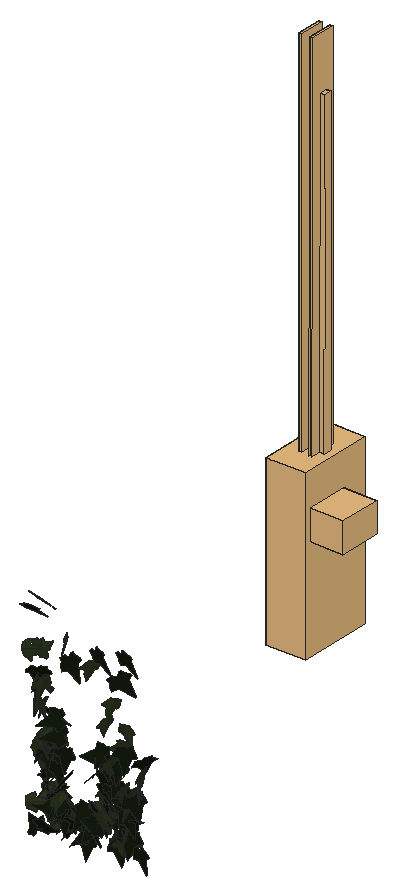
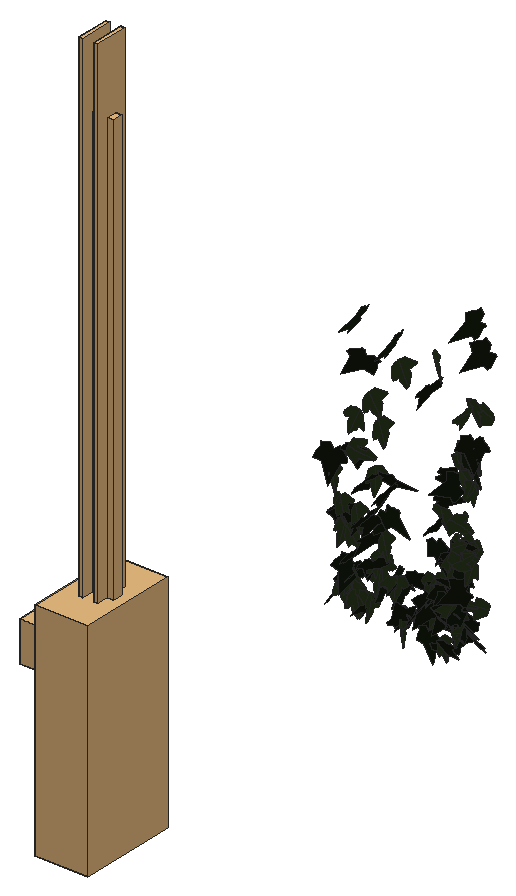
# SketchUp Ruby script. Lengths in inches.
U = 1.inch
M = Sketchup.active_model
def pt(a) = Geom::Point3d.new(a.map { |v| v * U })
def face(e, loops, mat)
  f = e.add_face(loops[0].map { |a| pt(a) })
  loops[1..].each { |l| e.add_face(l.map { |a| pt(a) }).erase! }
  f.material = f.back_material = mat if mat
  f
end
# faces: each face lists its corners as indices into pts; further lists are holes
def faces(e, pts, list, mat = nil) = list.each { |f| face(e, (f[0].is_a?(Array) ? f : [f]).map { |l| l.map { |i| pts[i] } }, mat) }
# xy, xz, yz: faces in a plane at the given z, y or x. An outline is a flat list of corners, or four numbers for a rectangle; further outlines are holes
def ring(l) = l.size == 4 ? [[l[0], l[1]], [l[2], l[1]], [l[2], l[3]], [l[0], l[3]]] : l.each_slice(2).to_a
def flat(e, list, mat, &to3) = list.each { |f| face(e, (f[0].is_a?(Array) ? f : [f]).map { |l| ring(l).map { |u, v| to3.(u, v) } }, mat) }
def xy(e, z, list, mat = nil) = flat(e, list, mat) { |x, y| [x, y, z] }
def xz(e, y, list, mat = nil) = flat(e, list, mat) { |x, z| [x, y, z] }
def yz(e, x, list, mat = nil) = flat(e, list, mat) { |y, z| [x, y, z] }
def lines(e, pts, list) = list.each { |a, b| e.add_line(pt(pts[a]), pt(pts[b])) }
# prism: a flat outline (further loops are holes) pulled along v
def prism(e, loops, v, mat = nil)
  f = face(e, loops, mat); d = Geom::Vector3d.new(v.map { |x| x * U })
  f.pushpull(f.normal.samedirection?(d) ? d.length : -d.length)
end
def box(e, o, s, mat = nil) = prism(e, [[o, [o[0] + s[0], o[1], o[2]], [o[0] + s[0], o[1] + s[1], o[2]], [o[0], o[1] + s[1], o[2]]]], [0, 0, s[2]], mat)
def at(x, y, z, deg = 0) = Geom::Transformation.translation(pt([x, y, z])) * Geom::Transformation.rotation(ORIGIN, Z_AXIS, deg.degrees)
def axes(o, x, y, z) = Geom::Transformation.new([*x, 0, *y, 0, *z, 0, *pt(o).to_a, 1])
def part(name) = M.definitions.add(name)
# library, detail: a bought-in or finely detailed component or shape, given as its bounding box
def library(name, o, s) = part(name).tap { |d| box(d.entities, o, s) }
def detail(e, o, s) = box(e.add_group.entities, o, s)
def put(e, d, t, mat = nil) = e.add_instance(d, t).tap { |i| i.material = mat if mat }
def group(e, t, mat = nil) = e.add_group.tap { |g| g.transformation = t; g.material = mat if mat }.entities
root = M.entities
M.materials.add("Glass Rail Metal").color = [192, 192, 192]
M.materials.add("[Translucent Glass Tinted]").color = [8, 201, 241]
M.materials["[Translucent Glass Tinted]"].alpha = 0.48
M.materials.add("efeu1").color = [18, 25, 13]
M.materials.add("efeu2").color = [43, 57, 29]
c1 = part("ivyleaf_9")
p = [[1.54,2.16,1.25],[1.36,2.04,1.19],[-0.21,0.99,0.68],[-0.71,1.11,0.82],[-0.85,0.86,0.67],[-0.8,0.17,0.21],
  [-0.9,-0.01,0.1],[-0.67,-0.16,-0.02],[-0.08,-0.08,-0.05],[-0.03,-0.6,-0.4],[0.65,-0.88,-0.66],[0.83,-0.6,-0.49],
  [1.29,-0.42,-0.43],[1.8125,-0.07,-0.26],[1.21,0.44,0.15]]
faces(c1.entities,p,[[0,1,2,3,4,5,6,7,8,9,10,11,12,13,14]],"efeu1")
c2 = part("ivyleaf_10")
p = [[0,0.5,-0.03],[-0.0625,2.02,-0.43],[-0.19,2.01,-0.46],[-0.54,1.05,-0.29],[-0.52,0.625,-0.18],[-0.83,0.76,-0.28],
  [-1.16,0.64,-0.33],[-1.15,0.33,-0.24],[-0.77,-0.39,0.02],[-0.3,-0.51,0.16],[0.04,-0.48,0.23],[-0.02,2.01,-0.4375],
  [-0.06,2.01,-0.43],[0.04,-0.49,0.23],[0.67,-0.49,0.14],[1.38,0.36,-0.2],[1.375,0.51,-0.24],[0.81,0.65,-0.19],
  [0.62,0.59,-0.15],[0.6,1.09,-0.28],[0.5,1.23,-0.31]]
faces(c2.entities,p,[[0,1,2,3,4,5,6,7,8,9,10],[11,12,0,13,14,15,16,17,18,19,20]],"efeu2")
c3 = library("glass bracket3",[-2.83,-0.98,-1],[3.67,3.29,2])
c4 = library("Group\#46",[0,0,0],[50.8,6,878.92])
c5 = library("Group\#15",[0.69,0,0.79],[0.62,1.89,30.3])
c6 = library("Group\#43",[0,0,0],[50.8,6,878.92])
c7 = library("Group\#53",[0,0,0],[3.15,5.91,11.14])
put(root,c1,axes([518.76,128.71,270.52],[0.73335,-0.82739,-0.07933],[0.07062,0.16744,-1.09346],[0.82818,0.71837,0.16349]))
put(root,c1,axes([508.96,129.22,258.32],[-0.73907,-0.28461,0.64117],[-0.60461,-0.2589,-0.77055],[0.41505,-0.88394,0.01925]))
put(root,c1,axes([505.71,128.29,274.43],[1.10412,-0.17355,0.00871],[0.04756,0.24793,-1.08883],[0.16713,1.07596,0.2523]))
put(root,c2,axes([513.88,129,267.48],[-0.28227,-1.01753,0.27722],[-0.03621,-0.27746,-1.05527],[1.05399,-0.28204,0.03799]))
put(root,c2,axes([516.99,128.65,255.53],[-0.22277,-1.0028,-0.22556],[0.03318,0.22366,-1.02713],[1.02732,-0.22468,-0.01574]))
put(root,c2,axes([509.16,128.75,248.03],[0.33895,0.95653,-0.16425],[-0.20094,-0.10349,-1.03639],[-1.02758,0.33575,0.14849]))
put(root,c1,axes([509.7,129.3,247.28],[-0.88288,-0.4898,0.19327],[-0.14417,-0.13829,-0.98979],[0.5471,-0.82686,0.05106]))
put(root,c1,axes([509.53,129.25,245.82],[0.01955,-0.95938,0.0947],[0.00483,-0.09099,-0.99793],[1.04078,0.01845,0.00285]))
put(root,c2,axes([510.04,128.89,269.49],[0.60989,-0.91075,-0.05301],[-0.01169,0.05595,-1.09589],[0.91222,0.60963,0.02139]))
put(root,c1,axes([506.24,128.73,243.21],[0.53244,-0.18494,0.76957],[0.78135,-0.16562,-0.54434],[0.26085,0.87359,0.05971]))
put(root,c1,axes([509.93,128.92,246.58],[-0.91388,0.50314,-0.2297],[0.19303,-0.13147,-1.02361],[-0.56118,-0.8646,0.02197]))
put(root,c2,axes([516.17,129.01,260.7],[-0.07613,-1.0616,0.10446],[0.01558,-0.10582,-1.06408],[1.06661,-0.07423,0.02299]))
put(root,c1,axes([514.6875,128.83,269.47],[0.75757,-0.77519,-0.19052],[-0.05686,0.20959,-1.07887],[0.79623,0.75251,0.10423]))
put(root,c2,axes([519.01,128.84,260.71],[-1.0052,0.2156,-0.32106],[0.29146,-0.16535,-1.02357],[-0.25419,-1.04219,0.09598]))
put(root,c1,axes([514.1,129.59,245.81],[-0.65738,-0.79377,0.25529],[-0.12052,-0.23122,-1.02927],[0.82505,-0.66623,0.05306]))
put(root,c2,axes([504.96,128.62,246.02],[0.22266,-0.0161,-0.94755],[0.94219,0.27331,0.20028],[0.28427,-0.89326,0.07836]))
put(root,c2,axes([506.76,128.87,254.4],[-0.65316,0.72386,-0.13088],[0.08258,-0.1001,-0.98097],[-0.78919,-0.60957,0.00568]))
put(root,c2,axes([516.92,129.34,263.35],[-0.3207,-0.9462,0.41234],[-0.01464,-0.42757,-0.99254],[1.03204,-0.30009,0.11405]))
put(root,c2,axes([515.79,128.93,247.58],[-0.99595,0.08341,-0.22059],[0.21073,-0.11506,-0.99493],[-0.10588,-1.01357,0.09479]))
put(root,c1,axes([515.46,129.13,255.62],[-0.78114,0.26971,0.6486],[-0.66455,0.03054,-0.81305],[-0.22759,-1.01486,0.1479]))
put(root,c1,axes([515.29,129.05,251.34],[0.84604,-0.67912,0.01835],[0.01525,-0.01032,-1.08489],[0.6792,0.84618,0.0015]))
put(root,c1,axes([515.52,128.67,253.86],[0.75836,-0.50956,-0.60101],[-0.37926,0.49511,-0.89833],[0.69067,0.83138,0.16662]))
put(root,c1,axes([509.02,129.59,255.82],[-0.62408,-0.18442,0.76326],[-0.71289,-0.32869,-0.62642],[0.39962,-0.87436,0.0745]))
put(root,c1,axes([509.99,128.8125,250.79],[-0.36749,0.91471,-0.15469],[0.05626,-0.13932,-1.01499],[-0.99928,-0.34424,-0.00026]))
put(root,c1,axes([518.77,129.32,257.58],[-0.73748,-0.49811,-0.58047],[0.48116,0.3247,-0.88994],[0.5946,-0.88056,0.0002]))
put(root,c2,axes([503.87,129.2,266.02],[0.32529,-0.18619,-0.9766],[0.97258,-0.27888,0.35791],[-0.35078,-0.9459,0.08671]))
put(root,c1,axes([507.17,128.55,248.64],[-0.15352,0.88052,0.29835],[-0.03681,0.28506,-0.92752],[-0.99948,-0.14575,-0.01167]))
put(root,c1,axes([513.19,129.57,244.82],[0.48168,-0.76677,0.5409],[0.38793,-0.3909,-0.89958],[0.85442,0.60974,0.1035]))
put(root,c1,axes([512.57,129.75,247.12],[-0.81766,-0.66586,0.01126],[-0.00826,-0.00769,-1.05448],[0.66591,-0.8177,0.00074]))
put(root,c2,axes([506.3,129.7,259.64],[0.28617,-0.79006,0.53749],[0.18463,-0.48776,-0.86662],[1.00275,0.31528,0.00617]))
put(root,c1,axes([517.8,129.0625,267.0625],[-0.10809,-0.35572,-1.02995],[0.5617,0.8687,-0.35898],[0.93372,-0.56377,0.09672]))
put(root,c1,axes([505.76,128.83,242.59],[-0.03602,0.49112,0.79904],[-0.60292,0.5969,-0.42202],[-0.77868,-0.48489,0.2898]))
put(root,c2,axes([506.15,129.59,262.2],[-0.13474,-1.03985,0.2075],[0.02286,-0.21196,-1.0474],[1.0601,-0.1276,0.04895]))
put(root,c1,axes([504.26,128.85,272.14],[1.07639,0.14162,0.11916],[0.09234,0.19902,-1.02933],[-0.17372,0.98328,0.19118]))
put(root,c1,axes([519.84,129.47,251.38],[-0.26919,-0.81765,-0.59146],[0.24318,0.54154,-0.85932],[0.97941,-0.3592,0.0508]))
put(root,c1,axes([510.23,129.37,266.84],[0.27012,-0.92167,-0.51108],[-0.10495,0.50145,-0.95977],[1.04864,0.2876,0.03559]))
put(root,c1,axes([509.58,128.91,245.02],[0.93279,0.51284,-0.07704],[-0.07071,-0.03482,-1.04465],[-0.55513,0.86617,0.00361]))
put(root,c2,axes([518.68,129.52,257.74],[0.30599,0.17713,-1.00278],[-1.01535,-0.02668,-0.31454],[-0.07756,1.04809,0.16147]))
put(root,c1,axes([517.2,130.09,255.01],[-0.14461,-1.02549,0.18647],[-0.00133,-0.18807,-1.03535],[1.04231,-0.14252,0.02455]))
put(root,c1,axes([507.49,129.92,245.77],[-0.6914,0.09464,0.66822],[-0.6891,-0.25994,-0.62134],[0.13084,-0.86896,0.25865]))
put(root,c2,axes([510.15,129.42,247.38],[-0.93441,0.47797,-0.06146],[0.06324,-0.01621,-1.02788],[-0.51628,-0.86706,-0.01467]))
put(root,c1,axes([509.02,130.23,253.75],[-0.02735,-1.0253,0.17872],[0.02701,-0.17942,-1.02519],[1.04041,-0.0223,0.03131]))
put(root,c2,axes([508.98,129.22,244.85],[0.63698,0.60096,0.5701],[0.14931,0.5932,-0.83103],[-0.8657,0.54449,0.27615]))
put(root,c2,axes([505.37,129.62,266.9],[0.81921,-0.44131,-0.45466],[-0.37676,0.26829,-0.91115],[0.5551,0.83337,0.05256]))
put(root,c1,axes([507.82,130.125,251.24],[0.18293,-0.91464,0.06599],[0.00096,-0.06436,-0.96733],[0.99018,0.16904,-0.01126]))
put(root,c2,axes([504.79,129.98,259.35],[-0.14666,0.82408,-0.47353],[-0.0054,-0.46065,-0.86554],[-1.01681,-0.11642,0.0729]))
put(root,c1,axes([512.28,130.27,243.04],[-0.01752,-0.99155,0.12454],[-0.02793,-0.12402,-0.99138],[0.99895,-0.02086,-0.02553]))
put(root,c2,axes([518.6,130.21,249.74],[0.15325,-0.92037,0.46601],[0.11957,-0.45211,-0.93222],[1.02467,0.19041,0.03908]))
put(root,c2,axes([520.89,129.81,254.97],[0.21102,-1.0348,-0.11686],[0.0168,0.12261,-1.05532],[1.04125,0.20773,0.04071]))
put(root,c2,axes([518.05,129.93,251.87],[0.08153,-1.04614,-0.0366],[0.00107,0.0368,-1.0493],[1.04678,0.08144,0.00392]))
put(root,c1,axes([512.48,130.18,243.78],[-0.9715,0.24702,-0.02149],[-0.03589,-0.22609,-0.97616],[-0.24534,-0.94507,0.22791]))
put(root,c2,axes([504.76,129.91,262.35],[0.51133,-0.83041,-0.17849],[-0.10616,0.14149,-0.99401],[0.90963,0.48331,-0.01568]))
put(root,c1,axes([514.71,130.23,254.89],[0.20272,-1.02413,-0.08631],[-0.0045,0.08709,-1.04393],[1.02775,0.20238,0.01245]))
put(root,c2,axes([519.66,130.07,252.21],[0.04143,-1.05163,0.02218],[-0.03348,-0.0235,-1.05188],[1.05133,0.04069,-0.03437]))
put(root,c1,axes([518.72,130.37,245.57],[-0.42712,-0.89986,-0.20001],[0.05613,0.19464,-0.99557],[0.92011,-0.42959,-0.03211]))
put(root,c2,axes([515.48,130.01,247.48],[-0.86181,-0.5295,0.15653],[-0.13407,-0.0808,-1.01148],[0.53563,-0.87218,-0.00132]))
put(root,c2,axes([508.29,130.1,255.33],[1.01895,-0.12137,-0.02746],[-0.02697,0.01282,-0.98925],[0.13141,0.94376,0.0099]))
put(root,c1,axes([515.43,130.74,247.52],[0.0813,-0.77395,0.66392],[0.07404,-0.65978,-0.7782],[1.017,0.10991,0.00358]))
put(root,c2,axes([507.6,129.92,244.93],[0.52833,-0.65279,-0.42046],[-0.21607,0.35444,-0.84696],[0.80062,0.52642,0.04888]))
put(root,c1,axes([506.73,129.9,258.26],[0.95307,-0.17529,0.37982],[0.39869,-0.01252,-0.93393],[0.18017,0.95497,0.05748]))
put(root,c1,axes([517.07,130.17,251.57],[0.32929,-0.91008,-0.37758],[-0.05653,0.38001,-0.96522],[0.98367,0.32649,0.07093]))
put(root,c1,axes([520.97,129.63,256.75],[0.38021,0.99082,-0.14473],[-0.0394,-0.13989,-1.06118],[-1.00055,0.38202,-0.01321]))
put(root,c1,axes([512.32,130.12,243.88],[-0.81306,0.58648,0.01633],[-0.04904,-0.04012,-1.00064],[-0.58465,-0.81224,0.06122]))
put(root,c1,axes([514.32,130.28,253.04],[-0.65313,0.71302,-0.37936],[0.02187,-0.47209,-0.92496],[-0.80737,-0.58959,0.28184]))
put(root,c1,axes([507,130.64,251.78],[-0.54028,-0.79789,-0.02459],[0.01111,0.02146,-0.97942],[0.86203,-0.50036,-0.00279]))
put(root,c1,axes([519.375,130.4,251.21],[-0.66665,-0.45262,-0.66713],[0.57166,0.345,-0.80532],[0.56845,-0.87776,0.02749]))
put(root,c2,axes([504.79,130.33,258.76],[-0.70573,0.3914,-0.61027],[0.50647,-0.35645,-0.79037],[-0.56904,-0.80267,0.0534]))
put(root,c1,axes([504.91,129.96,263.36],[0.51956,0.72287,-0.45402],[-0.27846,-0.3527,-0.90287],[-0.86847,0.54554,0.01787]))
put(root,c2,axes([520,130.14,252.39],[-0.77347,0.70826,0.12326],[-0.20972,-0.04913,-1.03377],[-0.68763,-0.78169,0.17665]))
put(root,c1,axes([505.47,130.1,261.54],[-0.57354,0.80182,0.02035],[-0.01007,0.01729,-1.0002],[-0.86616,-0.53114,-0.00184]))
put(root,c2,axes([518.22,130.06,245.77],[0.28283,-0.85179,-0.48721],[0.10749,0.53088,-0.86575],[0.97538,0.18849,0.23668]))
put(root,c1,axes([509.66,129.875,245.41],[0.90681,0.46455,0.0102],[0.0012,0.01824,-0.99783],[-0.50182,0.8395,0.01604]))
put(root,c2,axes([504.72,130.15,252.16],[-0.43262,-0.24929,0.86718],[0.76985,0.43264,0.49066],[-0.53924,0.81765,0.00476]))
put(root,c2,axes([518.46,130.76,245.47],[-0.69874,-0.6287,0.40681],[-0.03492,-0.52844,-0.87666],[0.74803,-0.61195,0.33907]))
put(root,c2,axes([514.56,130.49,250.4],[0.09787,-1.03114,-0.01242],[-0.00181,0.01231,-1.03577],[1.03121,0.09788,-0.00064]))
put(root,c1,axes([519.79,130.7,243.58],[0.38989,-0.93612,0.00333],[-0.01495,-0.00984,-1.01392],[0.93601,0.38978,-0.01758]))
put(root,c2,axes([504.72,130.49,253.6],[0.5534,0.00055,0.83687],[0.86901,0.00988,-0.53288],[-0.00932,0.95393,0.00504]))
put(root,c2,axes([505.92,130.52,261.125],[-0.9754,0.07278,0.28799],[0.29814,-0.0217,0.94232],[0.08202,0.94439,-0.00054]))
put(root,c1,axes([515.68,130.3125,252.15],[0.21412,-0.80032,-0.63154],[-0.13394,0.61764,-0.82812],[1.01066,0.25141,0.02405]))
put(root,c1,axes([517.79,130.74,245.9],[0.27451,-0.98439,-0.09733],[-0.00618,0.0993,-1.02174],[0.98917,0.27381,0.02062]))
put(root,c1,axes([517.85,130.61,248.06],[0.26684,-0.95174,-0.29866],[-0.01607,0.30502,-0.98637],[0.99738,0.25955,0.06401]))
put(root,c2,axes([518.1,130.72,245.27],[-0.13822,0.8933,-0.48133],[-0.12004,-0.49676,-0.88747],[-1.0076,-0.06336,0.17176]))
put(root,c1,axes([505.68,130.88,253.27],[-0.90194,-0.38212,-0.11304],[0.12287,0.01238,-0.95441],[0.41109,-0.84208,0.03726]))
put(root,c1,axes([505.5625,131,243.18],[0.2356,-0.46354,0.79773],[0.3846,-0.67962,-0.53246],[0.88824,0.41722,0.01896]))
put(root,c1,axes([514.03,131.14,245.43],[0.152,-0.74203,0.67043],[0.26904,-0.62278,-0.7503],[0.96317,0.29106,0.10378]))
put(root,c1,axes([507.8,130.19,247.3],[0.5773,0.69456,-0.26873],[-0.16023,-0.21185,-0.91143],[-0.78415,0.55463,-0.0116]))
put(root,c1,axes([515.51,130.79,247.96],[-0.2666,-0.85622,-0.49563],[0.21267,0.45171,-0.89474],[0.96619,-0.33568,0.06019]))
put(root,c2,axes([519.1,130.3125,250.38],[-0.30876,-0.87098,-0.4879],[0.16206,0.46019,-0.92409],[0.98508,-0.34871,-0.0009]))
put(root,c2,axes([518.69,130.8,244.63],[-0.74369,-0.67808,0.16239],[-0.02619,-0.21009,-0.99721],[0.69676,-0.73165,0.13585]))
put(root,c1,axes([510.52,130.7,244.71],[0.5289,-0.81515,-0.27055],[-0.07967,0.26981,-0.96863],[0.85517,0.52928,0.07709]))
put(root,c1,axes([512.78,130.98,247.1],[0.58204,-0.79216,0.25625],[0.15376,-0.205,-0.983],[0.81826,0.602,0.00245]))
put(root,c1,axes([516.29,131.01,243.42],[0.05873,-0.99008,-0.17126],[0.0295,0.17318,-0.99104],[1.00435,0.05281,0.03913]))
put(root,c1,axes([505.875,131.23,246.56],[0.78542,-0.50554,-0.22986],[0.18898,-0.13547,0.92105],[-0.56512,-0.74792,-0.01146]))
put(root,c2,axes([517.3,130.91,243.86],[-0.66233,-0.76235,0.1255],[0.0534,-0.21008,-0.9943],[0.77077,-0.64054,0.17673]))
put(root,c2,axes([515.23,130.49,246.71],[-0.83649,0.5067,0.28852],[-0.2507,0.14299,-0.97796],[-0.52644,-0.87322,0.00728]))
put(root,c1,axes([515.64,130.64,250.4],[0.20452,-0.74911,-0.68119],[0.08285,0.705,-0.75042],[1.00912,0.09394,0.19967]))
put(root,c2,axes([506.89,130.76,251.54],[-0.09137,0.9309,-0.12397],[-0.00036,-0.11972,-0.97206],[-1.01358,-0.08387,0.01152]))
put(root,c2,axes([504.57,130.67,251.25],[-0.95363,0.32095,-0.05913],[0.06595,0.0016,-0.97681],[-0.34579,-0.88482,-0.02322]))
put(root,c2,axes([517.29,130.91,244.13],[-0.32522,-0.96677,0.02313],[-0.00756,-0.02186,-1.02],[0.96701,-0.3253,-0.00019]))
put(root,c2,axes([506.05,131.2,255.49],[0.40094,0.42435,-0.74963],[-0.72126,-0.32442,-0.55636],[-0.54389,0.74304,0.1852]))
put(root,c2,axes([505.47,130.23,266.04],[0.29521,0.03463,-0.96041],[0.23469,0.93361,0.1033],[0.97007,-0.23641,0.26728]))
put(root,c1,axes([509.38,130.65,242.88],[-0.1698,0.93445,0.0318],[0.00577,0.03191,-0.98543],[-1.00973,-0.15696,-0.01098]))
put(root,c2,axes([515.74,130.8,244.12],[0.08287,-0.88455,-0.49433],[0.06391,0.49955,-0.88318],[1.01128,0.04091,0.09633]))
put(root,c2,axes([517.61,130.82,245.37],[0.18304,-0.0135,1.0075],[-0.98697,0.20373,0.18204],[-0.20283,-1.00352,0.02341]))
put(root,c2,axes([505.6,131.47,251.61],[0.42278,0.40341,0.75194],[-0.54032,-0.52199,0.5846],[0.71248,-0.63524,-0.00286]))
put(root,c2,axes([512.77,131.05,247.14],[0.66969,0.75499,0.11689],[-0.06111,0.20788,-0.99257],[-0.76153,0.64725,0.18245]))
put(root,c1,axes([518.03,130.66,246.87],[0.62213,0.82066,-0.01773],[-0.1177,0.06716,-1.02102],[-0.81237,0.61874,0.13435]))
put(root,c1,axes([507.09,130.91,247.26],[0.00462,0.893,-0.03847],[-0.00241,-0.03698,-0.92873],[-0.96526,0.00436,0.00214]))
put(root,c2,axes([505.85,131.36,246.4],[0.91693,0.33119,-0.02119],[-0.01948,-0.00981,-0.94777],[-0.35783,0.8492,-0.00269]))
put(root,c2,axes([506.07,131.14,252.92],[-0.4676,0.21768,-0.8078],[-0.71953,0.40051,0.50296],[0.49117,0.79395,-0.03223]))
put(root,c2,axes([507.1,131.64,243.12],[0.07318,-0.88371,0.17647],[0.03946,-0.16732,-0.92144],[0.97104,0.0734,0.02414]))
put(root,c2,axes([511.79,131.42,243.26],[0.36412,-0.90729,-0.20859],[0.00044,0.22415,-0.97418],[0.93096,0.35475,0.08205]))
put(root,c1,axes([505.33,131.71,246.31],[-0.92893,0.24169,-0.01533],[0.00018,-0.05383,-0.92761],[-0.26151,-0.85856,0.05384]))
put(root,c1,axes([511.96,131.32,243.58],[-0.51958,-0.43373,0.73756],[0.56344,0.47597,0.67681],[-0.64394,0.76643,-0.00292]))
put(root,c1,axes([504.96,131.14,248.84],[0.77554,0.31799,0.47639],[0.4244,0.2413,-0.81489],[-0.42727,0.81686,0.05527]))
put(root,c1,axes([507.08,132.15,243.19],[-0.86534,-0.3451,0.04823],[-0.04657,-0.01711,-0.9073],[0.37316,-0.8024,-0.0014]))
put(root,c1,axes([504.86,131.91,247.18],[0.95439,-0.12832,-0.04043],[-0.0408,0.01031,-0.92867],[0.13894,0.88449,0.00496]))
put(root,c2,axes([505.9375,131.96,247.11],[0.47819,0.72748,0.289],[0.13177,0.2509,-0.88531],[-0.83065,0.4586,0.02593]))
put(root,c1,axes([506.68,132.32,245.66],[-0.86105,0.29936,0.22478],[-0.22735,0.05401,-0.88537],[-0.32761,-0.82428,0.02363]))
put(root,c2,axes([505.16,131.62,244.77],[-0.01385,0.39937,-0.84658],[0.01752,0.81408,0.41511],[0.9791,-0.00892,-0.01941]))
put(root,c1,axes([506.23,131.73,246.57],[0.56945,0.67572,0.25425],[0.12514,0.2193,-0.89031],[-0.76591,0.53823,0.04357]))
put(root,c3,axes([511.95,178.46,263.5625],[1.9,0,0],[0,1.9,0],[0,0,2.261]),"[Translucent Glass Tinted]")
put(root,c4,axes([506.55,179.56,248.78],[0,0.0748,0],[-0.0748,0,0.00001],[0.00001,0,0.08902]),"[Translucent Glass Tinted]")
put(root,c5,axes([507.3,179.56,248.78],[0,1.9,0],[-1.9,0,0.00031],[0.00026,0,2.261]),"Glass Rail Metal")
put(root,c6,axes([504.91,179.56,248.78],[0,0.0748,0],[-0.0748,0,0.00001],[0.00001,0,0.08902]),"[Translucent Glass Tinted]")
put(root,c7,axes([502.51,175.85,245.62],[1.9,0,0],[0,1.9,0],[0,0,2.261]),"[Translucent Glass Tinted]")
